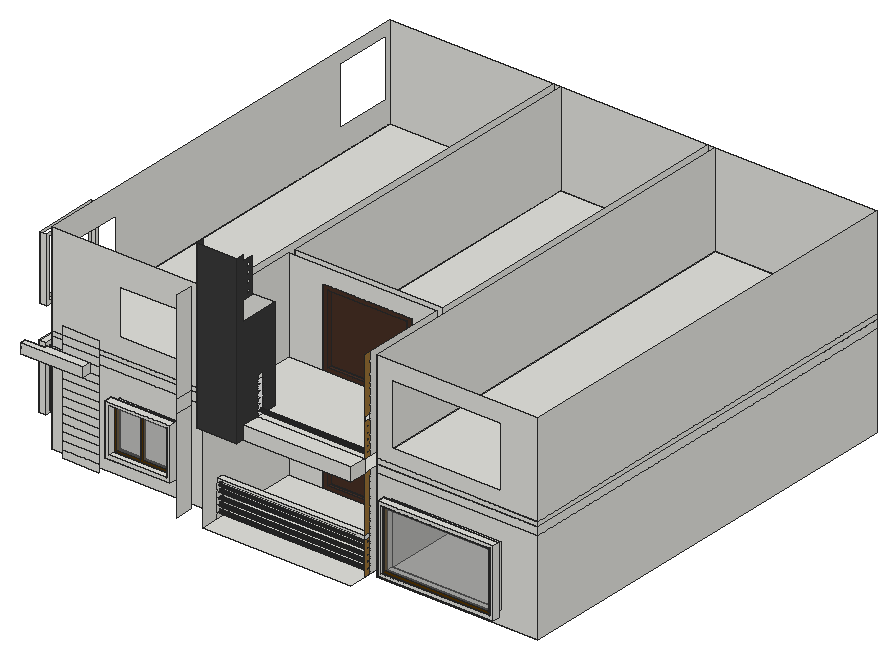
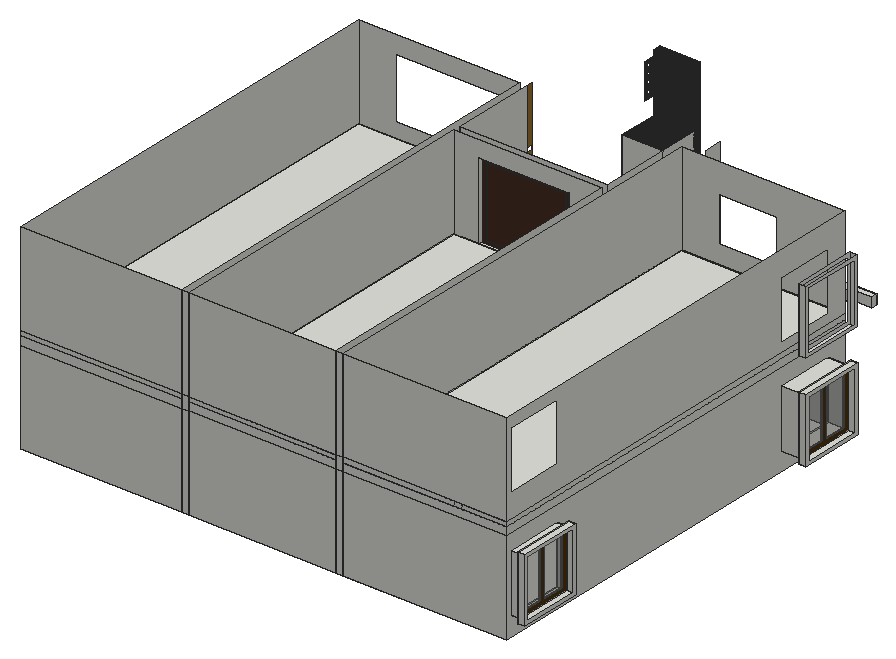
# SketchUp Ruby script. Lengths in inches.
U = 1.inch
M = Sketchup.active_model
def pt(a) = Geom::Point3d.new(a.map { |v| v * U })
def face(e, loops, mat)
  f = e.add_face(loops[0].map { |a| pt(a) })
  loops[1..].each { |l| e.add_face(l.map { |a| pt(a) }).erase! }
  f.material = f.back_material = mat if mat
  f
end
# faces: each face lists its corners as indices into pts; further lists are holes
def faces(e, pts, list, mat = nil) = list.each { |f| face(e, (f[0].is_a?(Array) ? f : [f]).map { |l| l.map { |i| pts[i] } }, mat) }
# xy, xz, yz: faces in a plane at the given z, y or x. An outline is a flat list of corners, or four numbers for a rectangle; further outlines are holes
def ring(l) = l.size == 4 ? [[l[0], l[1]], [l[2], l[1]], [l[2], l[3]], [l[0], l[3]]] : l.each_slice(2).to_a
def flat(e, list, mat, &to3) = list.each { |f| face(e, (f[0].is_a?(Array) ? f : [f]).map { |l| ring(l).map { |u, v| to3.(u, v) } }, mat) }
def xy(e, z, list, mat = nil) = flat(e, list, mat) { |x, y| [x, y, z] }
def xz(e, y, list, mat = nil) = flat(e, list, mat) { |x, z| [x, y, z] }
def yz(e, x, list, mat = nil) = flat(e, list, mat) { |y, z| [x, y, z] }
def lines(e, pts, list) = list.each { |a, b| e.add_line(pt(pts[a]), pt(pts[b])) }
# prism: a flat outline (further loops are holes) pulled along v
def prism(e, loops, v, mat = nil)
  f = face(e, loops, mat); d = Geom::Vector3d.new(v.map { |x| x * U })
  f.pushpull(f.normal.samedirection?(d) ? d.length : -d.length)
end
def box(e, o, s, mat = nil) = prism(e, [[o, [o[0] + s[0], o[1], o[2]], [o[0] + s[0], o[1] + s[1], o[2]], [o[0], o[1] + s[1], o[2]]]], [0, 0, s[2]], mat)
def at(x, y, z, deg = 0) = Geom::Transformation.translation(pt([x, y, z])) * Geom::Transformation.rotation(ORIGIN, Z_AXIS, deg.degrees)
def axes(o, x, y, z) = Geom::Transformation.new([*x, 0, *y, 0, *z, 0, *pt(o).to_a, 1])
def part(name) = M.definitions.add(name)
# library, detail: a bought-in or finely detailed component or shape, given as its bounding box
def library(name, o, s) = part(name).tap { |d| box(d.entities, o, s) }
def detail(e, o, s) = box(e.add_group.entities, o, s)
def put(e, d, t, mat = nil) = e.add_instance(d, t).tap { |i| i.material = mat if mat }
def group(e, t, mat = nil) = e.add_group.tap { |g| g.transformation = t; g.material = mat if mat }.entities
root = M.entities
M.materials.add("[Color C08]").color = [85, 51, 0]
M.materials.add("[Color D07]").color = [153, 114, 54]
M.materials.add("[Color M00]").color = [255, 255, 255]
M.materials.add("[Color M07]").color = [58, 58, 58]
M.materials.add("[Translucent Glass Gray]").color = [128, 128, 128]
M.materials["[Translucent Glass Gray]"].alpha = 0.5
M.materials.add("[Wood Veneer 01]").color = [71, 47, 37]
c1 = part("Group\#2")
xy(c1.entities,0,[[0,0,105.3125,8.625]],"[Wood Veneer 01]")
xy(c1.entities,6.5,[[6.5,0,98.81,8.625]],"[Wood Veneer 01]")
xy(c1.entities,132.37,[[6.5,0,98.81,8.625]],"[Wood Veneer 01]")
xy(c1.entities,138.875,[[0,0,105.3125,8.625]],"[Wood Veneer 01]")
xz(c1.entities,0,[[[0,0,105.3125,138.875],[6.5,6.5,98.81,132.37]]],"[Wood Veneer 01]")
xz(c1.entities,8.625,[[[0,0,105.3125,138.875],[6.5,6.5,98.81,132.37]],[6.5,6.5,98.81,132.37]],"[Wood Veneer 01]")
yz(c1.entities,0,[[0,0,8.625,138.875]],"[Wood Veneer 01]")
yz(c1.entities,6.5,[[0,6.5,8.625,132.37]],"[Wood Veneer 01]")
yz(c1.entities,98.81,[[0,6.5,8.625,132.37]],"[Wood Veneer 01]")
yz(c1.entities,105.3125,[[0,0,8.625,138.875]],"[Wood Veneer 01]")
c2 = part("Group\#3")
xy(c2.entities,0,[[0,0,69.125,3.25]],"[Color C08]")
xy(c2.entities,1.72,[[1.72,0,67.41,3.25]],"[Color C08]")
xy(c2.entities,48.28,[[1.72,0,67.41,3.25]],"[Color C08]")
xy(c2.entities,50,[[0,0,69.125,3.25]],"[Color C08]")
xz(c2.entities,0,[[[0,0,69.125,50],[1.72,1.72,67.41,48.28]]],"[Color C08]")
xz(c2.entities,0,[[1.72,1.72,67.41,48.28]],"[Translucent Glass Gray]")
xz(c2.entities,3.25,[[[0,0,69.125,50],[1.72,1.72,67.41,48.28]]],"[Color C08]")
yz(c2.entities,0,[[0,0,3.25,50]],"[Color C08]")
yz(c2.entities,1.72,[[0,1.72,3.25,48.28]],"[Color C08]")
yz(c2.entities,67.41,[[0,1.72,3.25,48.28]],"[Color C08]")
yz(c2.entities,69.125,[[0,0,3.25,50]],"[Color C08]")
c3 = part("Group\#4")
xy(c3.entities,0,[[0,0,0.4375,8.25]],"[Color C08]")
xy(c3.entities,9.875,[[0,0,0.4375,8.25]],"[Color C08]")
xz(c3.entities,0,[[0,0,0.4375,9.875]],"[Color C08]")
xz(c3.entities,0.45,[[0,0.45,0.4375,9.42]],"[Color C08]")
xz(c3.entities,4.05,[[0,0.49,0.4375,9.45]],"[Color C08]")
xz(c3.entities,4.38,[[0,0.49,0.4375,9.45]],"[Color C08]")
xz(c3.entities,7.8,[[0,0.45,0.4375,9.42]],"[Color C08]")
xz(c3.entities,8.25,[[0,0,0.4375,9.875]],"[Color C08]")
yz(c3.entities,0,[[[0,0,8.25,9.875],[0.45,0.45,4.05,0.49,4.05,9.45,0.45,9.42],[7.8,0.45,7.8,9.42,4.38,9.45,4.38,0.49]]],"[Color C08]")
yz(c3.entities,0,[[0.45,0.45,0.45,9.42,4.05,9.45,4.05,0.49],[7.8,0.45,4.38,0.49,4.38,9.45,7.8,9.42]],"[Translucent Glass Gray]")
yz(c3.entities,0.4375,[[[0,0,8.25,9.875],[0.45,0.45,0.45,9.42,4.05,9.45,4.05,0.49],[7.8,0.45,4.38,0.49,4.38,9.45,7.8,9.42]]],"[Color C08]")
p = [[0,4.05,0.49],[0,0.45,0.45],[0.4375,0.45,0.45],[0.4375,4.05,0.49],[0,7.8,0.45],[0,4.38,0.49],
  [0.4375,4.38,0.49],[0.4375,7.8,0.45],[0,0.45,9.42],[0,4.05,9.45],[0.4375,4.05,9.45],[0.4375,0.45,9.42],
  [0,4.38,9.45],[0,7.8,9.42],[0.4375,7.8,9.42],[0.4375,4.38,9.45]]
faces(c3.entities,p,[[0,1,2,3],[4,5,6,7],[8,9,10,11],[12,13,14,15]],"[Color C08]")
prism(root,[[[70.87,180.75,561.36],[95.94,180.75,561.36],[95.94,184.6875,561.36],[151.38,184.6875,561.36],[151.38,172.6875,561.36],[70.87,172.6875,561.36]]],[0,0,12.45])
xy(root,432,[[295.1875,187.375,486.25,187.375,486.25,326.375,453.82,326.375,453.82,335.375,338.07,335.375,338.07,326.375,295.1875,326.375],[75,218.375,286.1875,764.25],[495.25,218.375,703.3125,764.25],[295.1875,335.375,486.25,764.25]])
xy(root,446.34,[[510.53,200.375,659.59,209.375]])
xy(root,450.34,[[514.53,200.375,655.59,209.375],[514.53,209.375,655.59,218.375]])
xy(root,452.07,[[39.625,241.8125,48.625,325.0625]])
xy(root,453.91,[[54,679.03,63,761.4]])
xy(root,456.07,[[39.625,245.8125,48.625,321.0625],[48.625,245.8125,75,321.0625]])
xy(root,457.91,[[54,683.03,63,757.4],[63,683.03,75,757.4]])
xy(root,459.4,[[158.4,200.375,241.77,209.375]])
xy(root,463.4,[[162.4,200.375,237.77,209.375],[162.4,209.375,237.77,218.375]])
xy(root,475.1,[[295.1875,209.375,486.25,218.375]])
xy(root,480,[[295.1875,209.375,486.25,218.375]])
xy(root,521.59,[[162.4,200.375,237.77,209.375],[162.4,209.375,237.77,218.375]])
xy(root,525.59,[[158.4,200.375,241.77,209.375]])
xy(root,529.16,[[514.53,200.375,655.59,209.375],[514.53,209.375,655.59,218.375]])
xy(root,530.3125,[[338.07,326.375,453.82,335.375]])
xy(root,531.32,[[39.625,245.8125,48.625,321.0625],[48.625,245.8125,75,321.0625]])
xy(root,532.29,[[54,683.03,63,757.4],[63,683.03,75,757.4]])
xy(root,533.16,[[510.53,200.375,659.59,209.375]])
xy(root,535.32,[[39.625,241.8125,48.625,325.0625]])
xy(root,536.29,[[54,679.03,63,761.4]])
xy(root,552,[[295.1875,187.375,486.25,326.375]])
xy(root,552,[[295.1875,177.125,347.125,187.375]],"[Color M07]")
xy(root,563,[[75,218.375,286.1875,764.25],[495.25,218.375,703.3125,764.25],[295.1875,335.375,486.25,764.25]])
xy(root,569,[[295.1875,187.375,347.125,237.56],[347.125,187.375,486.25,210.1875],[347.125,210.1875,486.25,218.5625],[75,218.375,286.1875,764.25],[495.25,218.375,703.3125,764.25],
  [347.125,218.5625,486.25,218.5625,486.25,326.375,295.1875,326.375,295.1875,237.56,347.125,237.56],[338.07,326.375,453.82,335.375],[295.1875,335.375,486.25,764.25]])
xy(root,577.63,[[39.625,242.5625,48.625,325.8125]])
xz(root,177.125,[[295.1875,552,347.125,766]],"[Color M07]")
xz(root,187.375,[[295.1875,552,347.125,569],[347.125,552,486.25,569]])
xz(root,200.375,[[[510.53,446.34,659.59,533.16],[514.53,450.34,655.59,529.16]],[[158.4,459.4,241.77,525.59],[162.4,463.4,237.77,521.59]]])
xz(root,209.375,[[95.94,432.71,143.14,442.9],[95.94,442.9,143.14,453.09],[[510.53,446.34,659.59,533.16],[514.53,450.34,655.59,529.16]],[95.94,453.09,143.14,463.27],[[158.4,459.4,241.77,525.59],[162.4,463.4,237.77,521.59]],
  [95.94,463.27,143.14,473.46],[95.94,473.46,143.14,483.65],[295.1875,475.1,486.25,480],[95.94,483.65,143.14,493.84],[95.94,493.84,143.14,504.02],
  [95.94,504.02,143.14,514.21],[95.94,514.21,143.14,524.4],[95.94,524.4,143.14,534.59],[95.94,534.59,143.14,544.77],[95.94,544.77,143.14,554.96],
  [95.94,554.96,143.14,565.15],[95.94,565.15,143.14,575.34],[95.94,575.34,143.14,585.52]])
xz(root,218.375,[[[75,432,286.1875,552],[162.4,463.4,237.77,521.59]],[[495.25,432,703.3125,552],[514.53,450.34,655.59,529.16]],[295.1875,475.1,486.25,480],[75,552,286.1875,563],[495.25,552,703.3125,563],
  [75,563,286.1875,569],[495.25,563,703.3125,569],[[75,569,286.1875,689],[162.4,592.78,237.77,650.97]],[[495.25,569,703.3125,689],[514.53,587.28,655.59,666.09]]])
xz(root,237.56,[[295.1875,569,347.125,689]])
xz(root,241.8125,[[39.625,452.07,48.625,535.32]])
xz(root,242.5625,[[39.625,577.63,48.625,660.88]])
xz(root,245.8125,[[39.625,456.07,48.625,531.32],[48.625,456.07,75,531.32]])
xz(root,321.0625,[[39.625,456.07,48.625,531.32],[48.625,456.07,75,531.32]])
xz(root,325.0625,[[39.625,452.07,48.625,535.32]])
xz(root,325.8125,[[39.625,577.63,48.625,660.88]])
xz(root,326.375,[[295.1875,432,338.07,432,338.07,530.3125,453.82,530.3125,453.82,432,486.25,432,486.25,552,295.1875,552],[295.1875,569,338.07,569,338.07,668.5625,453.82,668.5625,453.82,569,486.25,569,486.25,689,295.1875,689]])
xz(root,335.375,[[295.1875,432,295.1875,552,486.25,552,486.25,432,453.82,432,453.82,530.3125,338.07,530.3125,338.07,432],[295.1875,552,486.25,563],[295.1875,563,476.48,569],[476.48,563,480.66,569],[480.66,563,486.25,569],
  [295.1875,569,295.1875,689,486.25,689,486.25,569,453.82,569,453.82,668.5625,338.07,668.5625,338.07,569]])
xz(root,679.03,[[54,453.91,63,536.29]])
xz(root,683.03,[[54,457.91,63,532.29],[63,457.91,75,532.29]])
xz(root,757.4,[[54,457.91,63,532.29],[63,457.91,75,532.29]])
xz(root,761.4,[[54,453.91,63,536.29]])
xz(root,764.25,[[75,432,286.1875,552],[286.1875,432,295.1875,552],[295.1875,432,486.25,552],[486.25,432,495.25,552],[495.25,432,703.3125,552],
  [75,552,286.1875,563],[286.1875,552,295.1875,569],[295.1875,552,486.25,563],[486.25,552,495.25,569],[495.25,552,703.3125,563],
  [75,563,133.66,569],[133.66,563,143.35,569],[143.35,563,286.1875,569],[295.1875,563,486.25,569],[495.25,563,703.3125,569],
  [75,569,286.1875,689],[286.1875,569,295.1875,689],[295.1875,569,486.25,689],[486.25,569,495.25,689],[495.25,569,703.3125,689]])
yz(root,39.625,[[[241.8125,452.07,325.0625,535.32],[245.8125,456.07,321.0625,531.32]],[[242.5625,577.63,325.8125,660.88],[246.5625,581.63,321.8125,656.88]]])
yz(root,48.625,[[[241.8125,452.07,325.0625,535.32],[245.8125,456.07,321.0625,531.32]],[[242.5625,577.63,325.8125,660.88],[246.5625,581.63,321.8125,656.88]]])
yz(root,54,[[[679.03,453.91,761.4,536.29],[683.03,457.91,757.4,532.29]]])
yz(root,63,[[[679.03,453.91,761.4,536.29],[683.03,457.91,757.4,532.29]]])
yz(root,75,[[[218.375,432,764.25,552],[245.8125,456.07,321.0625,531.32],[683.03,457.91,757.4,532.29]],[218.375,552,764.25,563],[218.375,563,764.25,569],[[218.375,569,764.25,689],[246.5625,581.63,321.8125,656.88],[683.03,599.54,757.4,673.91]]])
yz(root,158.4,[[200.375,459.4,209.375,525.59]])
yz(root,162.4,[[200.375,463.4,209.375,521.59],[209.375,463.4,218.375,521.59]])
yz(root,237.77,[[200.375,463.4,209.375,521.59],[209.375,463.4,218.375,521.59]])
yz(root,241.77,[[200.375,459.4,209.375,525.59]])
yz(root,261.34,[[187.375,432,209.375,552],[187.375,552,209.375,569],[187.375,569,209.375,689]])
yz(root,286.1875,[[218.375,432,764.25,552],[218.375,552,764.25,563],[218.375,563,764.25,569],[218.375,569,764.25,689]])
yz(root,295.1875,[[187.375,432,209.375,432,209.375,480,218.375,480,218.375,432,326.375,432,326.375,552,187.375,552],[[209.375,432,218.375,475.1],[213.95,437.92,213.5,437.98,213.07,438.15,212.71,438.43,212.43,438.79,212.26,439.21,212.2,439.67,212.26,440.12,212.43,440.54,212.71,440.9,213.07,441.18,213.5,441.36,213.95,441.42,214.4,441.36,214.82,441.18,215.1875,440.9,215.46,440.54,215.64,440.12,215.7,439.67,215.64,439.21,215.46,438.79,215.1875,438.43,214.82,438.15,214.4,437.98],[213.95,446.17,213.5,446.23,213.07,446.4,212.71,446.68,212.43,447.04,212.26,447.46,212.2,447.92,212.26,448.37,212.43,448.79,212.71,449.15,213.07,449.43,213.5,449.61,213.95,449.67,214.4,449.61,214.82,449.43,215.1875,449.15,215.46,448.79,215.64,448.37,215.7,447.92,215.64,447.46,215.46,447.04,215.1875,446.68,214.82,446.4,214.4,446.23],[213.95,453.92,213.5,453.98,213.07,454.15,212.71,454.43,212.43,454.79,212.26,455.21,212.2,455.67,212.26,456.12,212.43,456.54,212.71,456.9,213.07,457.18,213.5,457.36,213.95,457.42,214.4,457.36,214.82,457.18,215.1875,456.9,215.46,456.54,215.64,456.12,215.7,455.67,215.64,455.21,215.46,454.79,215.1875,454.43,214.82,454.15,214.4,453.98],[213.95,461.6,213.5,461.66,213.07,461.84,212.71,462.12,212.43,462.48,212.26,462.9,212.2,463.35,212.26,463.81,212.43,464.23,212.71,464.59,213.07,464.87,213.5,465.04,213.95,465.1,214.4,465.04,214.82,464.87,215.1875,464.59,215.46,464.23,215.64,463.81,215.7,463.35,215.64,462.9,215.46,462.48,215.1875,462.12,214.82,461.84,214.4,461.66],[213.95,469.3,213.5,469.36,213.07,469.54,212.71,469.8125,212.43,470.18,212.26,470.6,212.2,471.05,212.26,471.5,212.43,471.93,212.71,472.29,213.07,472.57,213.5,472.74,213.95,472.8,214.4,472.74,214.82,472.57,215.1875,472.29,215.46,471.93,215.64,471.5,215.7,471.05,215.64,470.6,215.46,470.18,215.1875,469.8125,214.82,469.54,214.4,469.36]],[335.375,432,764.25,552],[213.95,437.92,213.5,437.98,213.07,438.15,212.71,438.43,212.43,438.79,212.26,439.21,212.2,439.67,212.26,440.12,212.43,440.54,212.71,440.9,213.07,441.18,213.5,441.36,213.95,441.42,214.4,441.36,214.82,441.18,215.1875,440.9,215.46,440.54,215.64,440.12,215.7,439.67,215.64,439.21,215.46,438.79,215.1875,438.43,214.82,438.15,214.4,437.98],[213.95,446.17,213.5,446.23,213.07,446.4,212.71,446.68,212.43,447.04,212.26,447.46,212.2,447.92,212.26,448.37,212.43,448.79,212.71,449.15,213.07,449.43,213.5,449.61,213.95,449.67,214.4,449.61,214.82,449.43,215.1875,449.15,215.46,448.79,215.64,448.37,215.7,447.92,215.64,447.46,215.46,447.04,215.1875,446.68,214.82,446.4,214.4,446.23],
  [213.95,453.92,213.5,453.98,213.07,454.15,212.71,454.43,212.43,454.79,212.26,455.21,212.2,455.67,212.26,456.12,212.43,456.54,212.71,456.9,213.07,457.18,213.5,457.36,213.95,457.42,214.4,457.36,214.82,457.18,215.1875,456.9,215.46,456.54,215.64,456.12,215.7,455.67,215.64,455.21,215.46,454.79,215.1875,454.43,214.82,454.15,214.4,453.98],[213.95,461.6,213.5,461.66,213.07,461.84,212.71,462.12,212.43,462.48,212.26,462.9,212.2,463.35,212.26,463.81,212.43,464.23,212.71,464.59,213.07,464.87,213.5,465.04,213.95,465.1,214.4,465.04,214.82,464.87,215.1875,464.59,215.46,464.23,215.64,463.81,215.7,463.35,215.64,462.9,215.46,462.48,215.1875,462.12,214.82,461.84,214.4,461.66],[213.95,469.3,213.5,469.36,213.07,469.54,212.71,469.8125,212.43,470.18,212.26,470.6,212.2,471.05,212.26,471.5,212.43,471.93,212.71,472.29,213.07,472.57,213.5,472.74,213.95,472.8,214.4,472.74,214.82,472.57,215.1875,472.29,215.46,471.93,215.64,471.5,215.7,471.05,215.64,470.6,215.46,470.18,215.1875,469.8125,214.82,469.54,214.4,469.36],[209.375,475.1,218.375,480],[335.375,552,764.25,563],
  [335.375,563,764.25,569],[187.375,569,237.56,689],[237.56,569,326.375,689],[335.375,569,764.25,689]])
yz(root,295.1875,[[177.125,552,187.375,766]],"[Color M07]")
yz(root,338.07,[[326.375,432,335.375,530.3125],[326.375,569,335.375,668.5625]])
yz(root,347.125,[[[210.1875,569,218.5625,611.09],[214.5,573.16,214.95,573.22,215.375,573.39,215.74,573.67,216.01,574.03,216.1875,574.45,216.25,574.91,216.1875,575.36,216.01,575.78,215.74,576.14,215.375,576.42,214.95,576.6,214.5,576.66,214.05,576.6,213.625,576.42,213.26,576.14,212.98,575.78,212.81,575.36,212.75,574.91,212.81,574.45,212.98,574.03,213.26,573.67,213.625,573.39,214.05,573.22],[214.58,579.9,215.04,579.96,215.46,580.13,215.82,580.41,216.1,580.77,216.28,581.19,216.33,581.65,216.28,582.1,216.1,582.52,215.82,582.88,215.46,583.16,215.04,583.34,214.58,583.4,214.13,583.34,213.71,583.16,213.35,582.88,213.07,582.52,212.89,582.1,212.83,581.65,212.89,581.19,213.07,580.77,213.35,580.41,213.71,580.13,214.13,579.96],[214.58,587.58,215.04,587.64,215.46,587.82,215.82,588.1,216.1,588.46,216.28,588.88,216.33,589.33,216.28,589.79,216.1,590.21,215.82,590.57,215.46,590.85,215.04,591.03,214.58,591.08,214.13,591.03,213.71,590.85,213.35,590.57,213.07,590.21,212.89,589.79,212.83,589.33,212.89,588.88,213.07,588.46,213.35,588.1,213.71,587.82,214.13,587.64],[214.58,595.15,215.04,595.21,215.46,595.38,215.82,595.66,216.1,596.02,216.28,596.44,216.33,596.9,216.28,597.35,216.1,597.77,215.82,598.13,215.46,598.41,215.04,598.59,214.58,598.65,214.13,598.59,213.71,598.41,213.35,598.13,213.07,597.77,212.89,597.35,212.83,596.9,212.89,596.44,213.07,596.02,213.35,595.66,213.71,595.38,214.13,595.21],[214.41,603.03,214.86,603.09,215.28,603.26,215.64,603.54,215.92,603.9,216.1,604.32,216.16,604.78,216.1,605.23,215.92,605.65,215.64,606.02,215.28,606.29,214.86,606.47,214.41,606.53,213.95,606.47,213.53,606.29,213.17,606.02,212.89,605.65,212.72,605.23,212.66,604.78,212.72,604.32,212.89,603.9,213.17,603.54,213.53,603.26,213.95,603.09]],[214.5,573.16,214.05,573.22,213.625,573.39,213.26,573.67,212.98,574.03,212.81,574.45,212.75,574.91,212.81,575.36,212.98,575.78,213.26,576.14,213.625,576.42,214.05,576.6,214.5,576.66,214.95,576.6,215.375,576.42,215.74,576.14,216.01,575.78,216.1875,575.36,216.25,574.91,216.1875,574.45,216.01,574.03,215.74,573.67,215.375,573.39,214.95,573.22]],"[Color M00]")
yz(root,347.125,[[[177.125,552,177.125,766,187.375,766,187.375,758.77,201.8125,758.77,201.8125,713,187.375,713,187.375,689,237.56,689,237.56,569,218.5625,569,218.5625,617,210.1875,617,210.1875,569,187.375,569,187.375,552],[195.35,729.08,196.01,729.17,196.63,729.42,197.16,729.83,197.57,730.36,197.83,730.98,197.91,731.64,197.83,732.3,197.57,732.92,197.16,733.45,196.63,733.86,196.01,734.12,195.35,734.2,194.6875,734.12,194.07,733.86,193.54,733.45,193.13,732.92,192.875,732.3,192.79,731.64,192.875,730.98,193.13,730.36,193.54,729.83,194.07,729.42,194.6875,729.17],[195.35,739.2,196.01,739.29,196.63,739.55,197.16,739.95,197.57,740.48,197.83,741.1,197.91,741.77,197.83,742.43,197.57,743.05,197.16,743.58,196.63,743.98,196.01,744.24,195.35,744.33,194.6875,744.24,194.07,743.98,193.54,743.58,193.13,743.05,192.875,742.43,192.79,741.77,192.875,741.1,193.13,740.48,193.54,739.95,194.07,739.55,194.6875,739.29],[195.35,748.77,196.01,748.85,196.63,749.11,197.16,749.52,197.57,750.05,197.83,750.66,197.91,751.33,197.83,751.99,197.57,752.61,197.16,753.14,196.63,753.55,196.01,753.8,195.35,753.89,194.6875,753.8,194.07,753.55,193.54,753.14,193.13,752.61,192.875,751.99,192.79,751.33,192.875,750.66,193.13,750.05,193.54,749.52,194.07,749.11,194.6875,748.85],[195.35,717.83,196.01,717.92,196.63,718.17,197.16,718.58,197.57,719.11,197.83,719.73,197.91,720.39,197.83,721.05,197.57,721.67,197.16,722.2,196.63,722.61,196.01,722.87,195.35,722.95,194.6875,722.87,194.07,722.61,193.54,722.2,193.13,721.67,192.875,721.05,192.79,720.39,192.875,719.73,193.13,719.11,193.54,718.58,194.07,718.17,194.6875,717.92]]],"[Color M07]")
yz(root,453.82,[[326.375,432,335.375,530.3125],[326.375,569,335.375,668.5625]])
yz(root,486.25,[[218.375,432,326.375,552],[335.375,432,764.25,552],[209.375,475.1,218.375,480],[187.375,552,209.375,569],[335.375,552,764.25,563],
  [335.375,563,764.25,569],[218.375,569,218.375,611.09,218.5625,611.09,218.5625,617,218.375,617,218.375,689,326.375,689,326.375,569],[335.375,569,764.25,689]])
yz(root,486.25,[[[209.375,432,218.375,475.1],[213.95,461.6,214.4,461.66,214.82,461.84,215.1875,462.12,215.46,462.48,215.64,462.9,215.7,463.35,215.64,463.81,215.46,464.23,215.1875,464.59,214.82,464.87,214.4,465.04,213.95,465.1,213.5,465.04,213.07,464.87,212.71,464.59,212.43,464.23,212.26,463.81,212.2,463.35,212.26,462.9,212.43,462.48,212.71,462.12,213.07,461.84,213.5,461.66],[213.95,453.92,214.4,453.98,214.82,454.15,215.1875,454.43,215.46,454.79,215.64,455.21,215.7,455.67,215.64,456.12,215.46,456.54,215.1875,456.9,214.82,457.18,214.4,457.36,213.95,457.42,213.5,457.36,213.07,457.18,212.71,456.9,212.43,456.54,212.26,456.12,212.2,455.67,212.26,455.21,212.43,454.79,212.71,454.43,213.07,454.15,213.5,453.98],[213.95,446.17,214.4,446.23,214.82,446.4,215.1875,446.68,215.46,447.04,215.64,447.46,215.7,447.92,215.64,448.37,215.46,448.79,215.1875,449.15,214.82,449.43,214.4,449.61,213.95,449.67,213.5,449.61,213.07,449.43,212.71,449.15,212.43,448.79,212.26,448.37,212.2,447.92,212.26,447.46,212.43,447.04,212.71,446.68,213.07,446.4,213.5,446.23],[213.95,437.92,214.4,437.98,214.82,438.15,215.1875,438.43,215.46,438.79,215.64,439.21,215.7,439.67,215.64,440.12,215.46,440.54,215.1875,440.9,214.82,441.18,214.4,441.36,213.95,441.42,213.5,441.36,213.07,441.18,212.71,440.9,212.43,440.54,212.26,440.12,212.2,439.67,212.26,439.21,212.43,438.79,212.71,438.43,213.07,438.15,213.5,437.98],[213.95,469.3,214.4,469.36,214.82,469.54,215.1875,469.8125,215.46,470.18,215.64,470.6,215.7,471.05,215.64,471.5,215.46,471.93,215.1875,472.29,214.82,472.57,214.4,472.74,213.95,472.8,213.5,472.74,213.07,472.57,212.71,472.29,212.43,471.93,212.26,471.5,212.2,471.05,212.26,470.6,212.43,470.18,212.71,469.8125,213.07,469.54,213.5,469.36]],[209.375,480,218.375,552],[[209.375,569,209.375,689,218.375,689,218.375,617,210.1875,617,210.1875,611.09,218.375,611.09,218.375,569],[214.5,573.16,214.95,573.22,215.375,573.39,215.74,573.67,216.01,574.03,216.1875,574.45,216.25,574.91,216.1875,575.36,216.01,575.78,215.74,576.14,215.375,576.42,214.95,576.6,214.5,576.66,214.05,576.6,213.625,576.42,213.26,576.14,212.98,575.78,212.81,575.36,212.75,574.91,212.81,574.45,212.98,574.03,213.26,573.67,213.625,573.39,214.05,573.22],[214.58,587.58,215.04,587.64,215.46,587.82,215.82,588.1,216.1,588.46,216.28,588.88,216.33,589.33,216.28,589.79,216.1,590.21,215.82,590.57,215.46,590.85,215.04,591.03,214.58,591.08,214.13,591.03,213.71,590.85,213.35,590.57,213.07,590.21,212.89,589.79,212.83,589.33,212.89,588.88,213.07,588.46,213.35,588.1,213.71,587.82,214.13,587.64],[214.41,603.03,214.86,603.09,215.28,603.26,215.64,603.54,215.92,603.9,216.1,604.32,216.16,604.78,216.1,605.23,215.92,605.65,215.64,606.02,215.28,606.29,214.86,606.47,214.41,606.53,213.95,606.47,213.53,606.29,213.17,606.02,212.89,605.65,212.72,605.23,212.66,604.78,212.72,604.32,212.89,603.9,213.17,603.54,213.53,603.26,213.95,603.09],[214.58,579.9,215.04,579.96,215.46,580.13,215.82,580.41,216.1,580.77,216.28,581.19,216.33,581.65,216.28,582.1,216.1,582.52,215.82,582.88,215.46,583.16,215.04,583.34,214.58,583.4,214.13,583.34,213.71,583.16,213.35,582.88,213.07,582.52,212.89,582.1,212.83,581.65,212.89,581.19,213.07,580.77,213.35,580.41,213.71,580.13,214.13,579.96],[214.58,595.15,215.04,595.21,215.46,595.38,215.82,595.66,216.1,596.02,216.28,596.44,216.33,596.9,216.28,597.35,216.1,597.77,215.82,598.13,215.46,598.41,215.04,598.59,214.58,598.65,214.13,598.59,213.71,598.41,213.35,598.13,213.07,597.77,212.89,597.35,212.83,596.9,212.89,596.44,213.07,596.02,213.35,595.66,213.71,595.38,214.13,595.21]]],"[Color D07]")
yz(root,495.25,[[218.375,432,764.25,552],[218.375,552,764.25,563],[218.375,563,240.65,569],[240.65,563,260.59,569],[260.59,563,764.25,569],
  [218.375,569,764.25,689]])
yz(root,510.53,[[200.375,446.34,209.375,533.16]])
yz(root,514.53,[[200.375,450.34,209.375,529.16],[209.375,450.34,218.375,529.16]])
yz(root,655.59,[[200.375,450.34,209.375,529.16],[209.375,450.34,218.375,529.16]])
yz(root,659.59,[[200.375,446.34,209.375,533.16]])
yz(root,703.3125,[[218.375,432,764.25,552],[218.375,552,764.25,563],[218.375,563,764.25,569],[218.375,569,764.25,689]])
p = [[295.1875,213.5,437.98],[295.1875,213.95,437.92],[486.25,213.95,437.92],[486.25,213.5,437.98],[295.1875,214.4,437.98],[486.25,214.4,437.98],
  [295.1875,213.07,438.15],[486.25,213.07,438.15],[295.1875,214.82,438.15],[486.25,214.82,438.15],[295.1875,212.71,438.43],[486.25,212.71,438.43],
  [295.1875,215.1875,438.43],[486.25,215.1875,438.43],[295.1875,212.43,438.79],[486.25,212.43,438.79],[295.1875,215.46,438.79],[486.25,215.46,438.79],
  [295.1875,212.26,439.21],[486.25,212.26,439.21],[295.1875,215.64,439.21],[486.25,215.64,439.21],[295.1875,212.2,439.67],[486.25,212.2,439.67],
  [295.1875,215.7,439.67],[486.25,215.7,439.67],[295.1875,212.26,440.12],[486.25,212.26,440.12],[295.1875,215.64,440.12],[486.25,215.64,440.12],
  [295.1875,212.43,440.54],[486.25,212.43,440.54],[295.1875,215.46,440.54],[486.25,215.46,440.54],[295.1875,212.71,440.9],[486.25,212.71,440.9],
  [295.1875,215.1875,440.9],[486.25,215.1875,440.9],[295.1875,213.07,441.18],[486.25,213.07,441.18],[295.1875,214.82,441.18],[486.25,214.82,441.18],
  [295.1875,213.5,441.36],[486.25,213.5,441.36],[295.1875,214.4,441.36],[486.25,214.4,441.36],[295.1875,213.95,441.42],[486.25,213.95,441.42],
  [295.1875,213.07,446.4],[295.1875,213.5,446.23],[486.25,213.5,446.23],[486.25,213.07,446.4],[295.1875,213.95,446.17],[486.25,213.95,446.17],
  [295.1875,214.4,446.23],[486.25,214.4,446.23],[295.1875,214.82,446.4],[486.25,214.82,446.4],[295.1875,212.71,446.68],[486.25,212.71,446.68],
  [295.1875,215.1875,446.68],[486.25,215.1875,446.68],[295.1875,212.43,447.04],[486.25,212.43,447.04],[295.1875,215.46,447.04],[486.25,215.46,447.04],
  [295.1875,212.26,447.46],[486.25,212.26,447.46],[295.1875,215.64,447.46],[486.25,215.64,447.46],[295.1875,212.2,447.92],[486.25,212.2,447.92],
  [295.1875,215.7,447.92],[486.25,215.7,447.92],[295.1875,212.26,448.37],[486.25,212.26,448.37],[295.1875,215.64,448.37],[486.25,215.64,448.37],
  [295.1875,212.43,448.79],[486.25,212.43,448.79],[295.1875,215.46,448.79],[486.25,215.46,448.79],[295.1875,212.71,449.15],[486.25,212.71,449.15],
  [295.1875,215.1875,449.15],[486.25,215.1875,449.15],[295.1875,213.07,449.43],[486.25,213.07,449.43],[295.1875,214.82,449.43],[486.25,214.82,449.43],
  [295.1875,213.5,449.61],[486.25,213.5,449.61],[295.1875,214.4,449.61],[486.25,214.4,449.61],[295.1875,213.95,449.67],[486.25,213.95,449.67],
  [295.1875,213.5,453.98],[295.1875,213.95,453.92],[486.25,213.95,453.92],[486.25,213.5,453.98],[295.1875,214.4,453.98],[486.25,214.4,453.98],
  [295.1875,213.07,454.15],[486.25,213.07,454.15],[295.1875,214.82,454.15],[486.25,214.82,454.15],[295.1875,212.71,454.43],[486.25,212.71,454.43],
  [295.1875,215.1875,454.43],[486.25,215.1875,454.43],[295.1875,212.43,454.79],[486.25,212.43,454.79],[295.1875,215.46,454.79],[486.25,215.46,454.79],
  [295.1875,212.26,455.21],[486.25,212.26,455.21],[295.1875,215.64,455.21],[486.25,215.64,455.21],[295.1875,212.2,455.67],[486.25,212.2,455.67],
  [295.1875,215.7,455.67],[486.25,215.7,455.67],[295.1875,212.26,456.12],[486.25,212.26,456.12],[295.1875,215.64,456.12],[486.25,215.64,456.12],
  [295.1875,212.43,456.54],[486.25,212.43,456.54],[295.1875,215.46,456.54],[486.25,215.46,456.54],[295.1875,212.71,456.9],[486.25,212.71,456.9],
  [295.1875,215.1875,456.9],[486.25,215.1875,456.9],[295.1875,213.07,457.18],[486.25,213.07,457.18],[295.1875,214.82,457.18],[486.25,214.82,457.18],
  [295.1875,213.5,457.36],[486.25,213.5,457.36],[295.1875,214.4,457.36],[486.25,214.4,457.36],[295.1875,213.95,457.42],[486.25,213.95,457.42],
  [295.1875,213.5,461.66],[295.1875,213.95,461.6],[486.25,213.95,461.6],[486.25,213.5,461.66],[295.1875,214.4,461.66],[486.25,214.4,461.66],
  [295.1875,213.07,461.84],[486.25,213.07,461.84],[295.1875,214.82,461.84],[486.25,214.82,461.84],[295.1875,212.71,462.12],[486.25,212.71,462.12],
  [295.1875,215.1875,462.12],[486.25,215.1875,462.12],[295.1875,212.43,462.48],[486.25,212.43,462.48],[295.1875,215.46,462.48],[486.25,215.46,462.48],
  [295.1875,212.26,462.9],[486.25,212.26,462.9],[295.1875,215.64,462.9],[486.25,215.64,462.9],[295.1875,212.2,463.35],[486.25,212.2,463.35],
  [295.1875,215.7,463.35],[486.25,215.7,463.35],[295.1875,212.26,463.81],[486.25,212.26,463.81],[295.1875,215.64,463.81],[486.25,215.64,463.81],
  [295.1875,212.43,464.23],[486.25,212.43,464.23],[295.1875,215.46,464.23],[486.25,215.46,464.23],[295.1875,212.71,464.59],[486.25,212.71,464.59],
  [295.1875,215.1875,464.59],[486.25,215.1875,464.59],[295.1875,213.07,464.87],[486.25,213.07,464.87],[295.1875,214.82,464.87],[486.25,214.82,464.87],
  [295.1875,213.5,465.04],[486.25,213.5,465.04],[295.1875,214.4,465.04],[486.25,214.4,465.04],[295.1875,213.95,465.1],[486.25,213.95,465.1],
  [295.1875,213.5,469.36],[295.1875,213.95,469.3],[486.25,213.95,469.3],[486.25,213.5,469.36],[295.1875,214.4,469.36],[486.25,214.4,469.36],
  [295.1875,213.07,469.54],[486.25,213.07,469.54],[295.1875,214.82,469.54],[486.25,214.82,469.54],[295.1875,212.71,469.8125],[486.25,212.71,469.8125],
  [295.1875,215.1875,469.8125],[486.25,215.1875,469.8125],[295.1875,212.43,470.18],[486.25,212.43,470.18],[295.1875,215.46,470.18],[486.25,215.46,470.18],
  [295.1875,212.26,470.6],[486.25,212.26,470.6],[295.1875,215.64,470.6],[486.25,215.64,470.6],[295.1875,212.2,471.05],[486.25,212.2,471.05],
  [295.1875,215.7,471.05],[486.25,215.7,471.05],[295.1875,212.26,471.5],[486.25,212.26,471.5],[295.1875,215.64,471.5],[486.25,215.64,471.5],
  [295.1875,212.43,471.93],[486.25,212.43,471.93],[295.1875,215.46,471.93],[486.25,215.46,471.93],[295.1875,212.71,472.29],[486.25,212.71,472.29],
  [295.1875,215.1875,472.29],[486.25,215.1875,472.29],[295.1875,213.07,472.57],[486.25,213.07,472.57],[295.1875,214.82,472.57],[486.25,214.82,472.57],
  [295.1875,213.5,472.74],[486.25,213.5,472.74],[295.1875,214.4,472.74],[486.25,214.4,472.74],[295.1875,213.95,472.8],[486.25,213.95,472.8],
  [347.125,213.625,573.39],[347.125,214.05,573.22],[486.25,214.05,573.22],[486.25,213.625,573.39],[347.125,214.5,573.16],[486.25,214.5,573.16],
  [347.125,214.95,573.22],[486.25,214.95,573.22],[347.125,215.375,573.39],[486.25,215.375,573.39],[347.125,213.26,573.67],[486.25,213.26,573.67],
  [347.125,215.74,573.67],[486.25,215.74,573.67],[347.125,212.98,574.03],[486.25,212.98,574.03],[347.125,216.01,574.03],[486.25,216.01,574.03],
  [347.125,212.81,574.45],[486.25,212.81,574.45],[347.125,216.1875,574.45],[486.25,216.1875,574.45],[347.125,212.75,574.91],[486.25,212.75,574.91],
  [347.125,216.25,574.91],[486.25,216.25,574.91],[347.125,212.81,575.36],[486.25,212.81,575.36],[347.125,216.1875,575.36],[486.25,216.1875,575.36],
  [347.125,212.98,575.78],[486.25,212.98,575.78],[347.125,216.01,575.78],[486.25,216.01,575.78],[347.125,213.26,576.14],[486.25,213.26,576.14],
  [347.125,215.74,576.14],[486.25,215.74,576.14],[347.125,213.625,576.42],[486.25,213.625,576.42],[347.125,215.375,576.42],[486.25,215.375,576.42],
  [347.125,214.05,576.6],[486.25,214.05,576.6],[347.125,214.95,576.6],[486.25,214.95,576.6],[347.125,214.5,576.66],[486.25,214.5,576.66]]
faces(root,p,[[0,1,2,3],[1,4,5,2],[6,0,3,7],[4,8,9,5],[10,6,7,11],[8,12,13,9],[14,10,11,15],[12,16,17,13],
  [18,14,15,19],[16,20,21,17],[22,18,19,23],[20,24,25,21],[26,22,23,27],[24,28,29,25],[30,26,27,31],[28,32,33,29],
  [34,30,31,35],[32,36,37,33],[38,34,35,39],[36,40,41,37],[42,38,39,43],[40,44,45,41],[46,42,43,47],[44,46,47,45],
  [48,49,50,51],[49,52,53,50],[52,54,55,53],[54,56,57,55],[58,48,51,59],[56,60,61,57],[62,58,59,63],[60,64,65,61],
  [66,62,63,67],[64,68,69,65],[70,66,67,71],[68,72,73,69],[74,70,71,75],[72,76,77,73],[78,74,75,79],[76,80,81,77],
  [82,78,79,83],[80,84,85,81],[86,82,83,87],[84,88,89,85],[90,86,87,91],[88,92,93,89],[94,90,91,95],[92,94,95,93],
  [96,97,98,99],[97,100,101,98],[102,96,99,103],[100,104,105,101],[106,102,103,107],[104,108,109,105],[110,106,107,111],[108,112,113,109],
  [114,110,111,115],[112,116,117,113],[118,114,115,119],[116,120,121,117],[122,118,119,123],[120,124,125,121],[126,122,123,127],[124,128,129,125],
  [130,126,127,131],[128,132,133,129],[134,130,131,135],[132,136,137,133],[138,134,135,139],[136,140,141,137],[142,138,139,143],[140,142,143,141],
  [144,145,146,147],[145,148,149,146],[150,144,147,151],[148,152,153,149],[154,150,151,155],[152,156,157,153],[158,154,155,159],[156,160,161,157],
  [162,158,159,163],[160,164,165,161],[166,162,163,167],[164,168,169,165],[170,166,167,171],[168,172,173,169],[174,170,171,175],[172,176,177,173],
  [178,174,175,179],[176,180,181,177],[182,178,179,183],[180,184,185,181],[186,182,183,187],[184,188,189,185],[190,186,187,191],[188,190,191,189],
  [192,193,194,195],[193,196,197,194],[198,192,195,199],[196,200,201,197],[202,198,199,203],[200,204,205,201],[206,202,203,207],[204,208,209,205],
  [210,206,207,211],[208,212,213,209],[214,210,211,215],[212,216,217,213],[218,214,215,219],[216,220,221,217],[222,218,219,223],[220,224,225,221],
  [226,222,223,227],[224,228,229,225],[230,226,227,231],[228,232,233,229],[234,230,231,235],[232,236,237,233],[238,234,235,239],[236,238,239,237]])
faces(root,p,[[240,241,242,243],[241,244,245,242],[244,246,247,245],[246,248,249,247],[250,240,243,251],[248,252,253,249],[254,250,251,255],[252,256,257,253],
  [258,254,255,259],[256,260,261,257],[262,258,259,263],[260,264,265,261],[266,262,263,267],[264,268,269,265],[270,266,267,271],[268,272,273,269],
  [274,270,271,275],[272,276,277,273],[278,274,275,279],[276,280,281,277],[282,278,279,283],[280,284,285,281],[286,282,283,287],[284,286,287,285]],"[Color M00]")
put(root,c1,axes([338.07,326.375,432],[1.09911,0,0],[0,0.6,0],[0,0,0.70792]))
put(root,c2,axes([514.53,202.875,450.34],[2.04069,0,0],[0,1,0],[0,0,1.57625]))
put(root,c3,axes([48.625,245.8125,456.07],[8.6376,0,0],[0,9.1053,0],[0,0,7.62025]))
put(root,c3,axes([63,683.03,457.91],[8.6376,0,0],[0,9.01515,0],[0,0,7.53165]))
put(root,c3,axes([237.77,209.375,463.4],[0,6.04632,0],[-9.13636,0,0],[0,0,5.89241]))
put(root,c1,axes([338.07,326.375,569],[1.09911,0,0],[0,0.6,0],[0,0,0.71692]))
